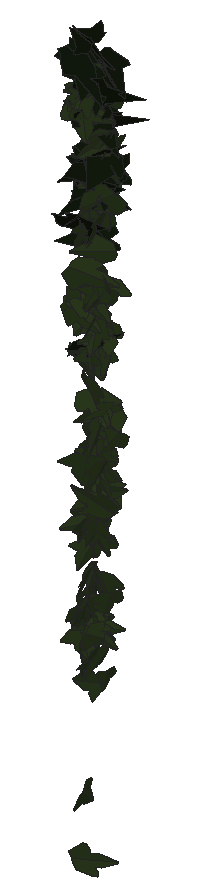
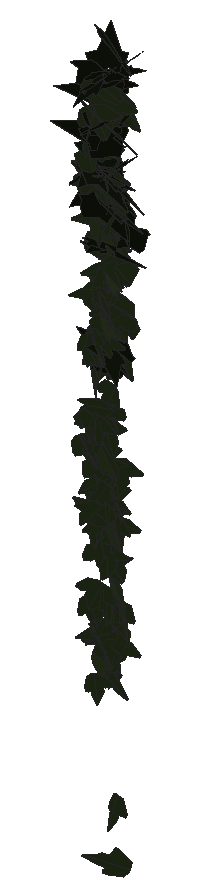
# SketchUp Ruby script. Lengths in inches.
U = 1.inch
M = Sketchup.active_model
def pt(a) = Geom::Point3d.new(a.map { |v| v * U })
def face(e, loops, mat)
  f = e.add_face(loops[0].map { |a| pt(a) })
  loops[1..].each { |l| e.add_face(l.map { |a| pt(a) }).erase! }
  f.material = f.back_material = mat if mat
  f
end
# faces: each face lists its corners as indices into pts; further lists are holes
def faces(e, pts, list, mat = nil) = list.each { |f| face(e, (f[0].is_a?(Array) ? f : [f]).map { |l| l.map { |i| pts[i] } }, mat) }
# xy, xz, yz: faces in a plane at the given z, y or x. An outline is a flat list of corners, or four numbers for a rectangle; further outlines are holes
def ring(l) = l.size == 4 ? [[l[0], l[1]], [l[2], l[1]], [l[2], l[3]], [l[0], l[3]]] : l.each_slice(2).to_a
def flat(e, list, mat, &to3) = list.each { |f| face(e, (f[0].is_a?(Array) ? f : [f]).map { |l| ring(l).map { |u, v| to3.(u, v) } }, mat) }
def xy(e, z, list, mat = nil) = flat(e, list, mat) { |x, y| [x, y, z] }
def xz(e, y, list, mat = nil) = flat(e, list, mat) { |x, z| [x, y, z] }
def yz(e, x, list, mat = nil) = flat(e, list, mat) { |y, z| [x, y, z] }
def lines(e, pts, list) = list.each { |a, b| e.add_line(pt(pts[a]), pt(pts[b])) }
# prism: a flat outline (further loops are holes) pulled along v
def prism(e, loops, v, mat = nil)
  f = face(e, loops, mat); d = Geom::Vector3d.new(v.map { |x| x * U })
  f.pushpull(f.normal.samedirection?(d) ? d.length : -d.length)
end
def box(e, o, s, mat = nil) = prism(e, [[o, [o[0] + s[0], o[1], o[2]], [o[0] + s[0], o[1] + s[1], o[2]], [o[0], o[1] + s[1], o[2]]]], [0, 0, s[2]], mat)
def at(x, y, z, deg = 0) = Geom::Transformation.translation(pt([x, y, z])) * Geom::Transformation.rotation(ORIGIN, Z_AXIS, deg.degrees)
def axes(o, x, y, z) = Geom::Transformation.new([*x, 0, *y, 0, *z, 0, *pt(o).to_a, 1])
def part(name) = M.definitions.add(name)
# library, detail: a bought-in or finely detailed component or shape, given as its bounding box
def library(name, o, s) = part(name).tap { |d| box(d.entities, o, s) }
def detail(e, o, s) = box(e.add_group.entities, o, s)
def put(e, d, t, mat = nil) = e.add_instance(d, t).tap { |i| i.material = mat if mat }
def group(e, t, mat = nil) = e.add_group.tap { |g| g.transformation = t; g.material = mat if mat }.entities
root = M.entities
M.materials.add("1026 AP 7946 SUNNY SIDE UP").color = [254, 231, 186]
M.materials.add("efeu1").color = [18, 25, 13]
M.materials.add("efeu2").color = [43, 57, 29]
c1 = part("ivyleaf_10")
p = [[0,0.5,-0.03],[-0.0625,2.02,-0.43],[-0.19,2.01,-0.46],[-0.54,1.05,-0.29],[-0.52,0.625,-0.18],[-0.83,0.76,-0.28],
  [-1.16,0.64,-0.33],[-1.15,0.33,-0.24],[-0.77,-0.39,0.02],[-0.3,-0.51,0.16],[0.04,-0.48,0.23],[-0.02,2.01,-0.4375],
  [-0.06,2.01,-0.43],[0.04,-0.49,0.23],[0.67,-0.49,0.14],[1.38,0.36,-0.2],[1.375,0.51,-0.24],[0.81,0.65,-0.19],
  [0.62,0.59,-0.15],[0.6,1.09,-0.28],[0.5,1.23,-0.31]]
faces(c1.entities,p,[[0,1,2,3,4,5,6,7,8,9,10],[11,12,0,13,14,15,16,17,18,19,20]],"efeu2")
c2 = part("ivyleaf_9")
p = [[1.54,2.16,1.25],[1.36,2.04,1.19],[-0.21,0.99,0.68],[-0.71,1.11,0.82],[-0.85,0.86,0.67],[-0.8,0.17,0.21],
  [-0.9,-0.01,0.1],[-0.67,-0.16,-0.02],[-0.08,-0.08,-0.05],[-0.03,-0.6,-0.4],[0.65,-0.88,-0.66],[0.83,-0.6,-0.49],
  [1.29,-0.42,-0.43],[1.8125,-0.07,-0.26],[1.21,0.44,0.15]]
faces(c2.entities,p,[[0,1,2,3,4,5,6,7,8,9,10,11,12,13,14]],"efeu1")
put(root,c1,axes([99.3125,212.71,264.43],[-0.12785,0.21743,0.05736],[-0.07153,0.0407,-0.23721],[-0.3451,-0.08899,0.02792]),"1026 AP 7946 SUNNY SIDE UP")
put(root,c1,axes([99.32,212.63,257.54],[0.10302,-0.18844,-0.06794],[-0.02315,0.06353,-0.20504],[0.31252,0.06682,0.0072]),"1026 AP 7946 SUNNY SIDE UP")
put(root,c1,axes([99.4,212.64,266.76],[0.25779,-0.12483,-0.10927],[-0.15343,0.04752,-0.20886],[0.22457,0.17576,-0.01726]),"1026 AP 7946 SUNNY SIDE UP")
put(root,c1,axes([99.25,212.95,264.75],[-0.09069,0.23059,-0.04473],[0.00337,-0.04554,-0.24497],[-0.36932,-0.05704,0.00875]),"1026 AP 7946 SUNNY SIDE UP")
put(root,c1,axes([99.33,212.89,258.47],[-0.11329,-0.16436,0.10325],[0.01129,-0.11018,-0.17981],[0.30326,-0.0573,0.04527]),"1026 AP 7946 SUNNY SIDE UP")
put(root,c2,axes([99.49,212.85,265.46],[-0.29653,0.15424,-0.02154],[0.00846,-0.02773,-0.25046],[-0.24478,-0.1878,0.01743]),"1026 AP 7946 SUNNY SIDE UP")
put(root,c2,axes([99.49,212.71,267.73],[-0.08229,0.16878,0.1343],[-0.09177,0.11209,-0.18553],[-0.34269,-0.07054,0.01743]),"1026 AP 7946 SUNNY SIDE UP")
put(root,c1,axes([99.32,212.84,265.11],[-0.32117,0.13465,-0.01253],[0.00024,-0.02319,-0.25138],[-0.2127,-0.20334,0.01864]),"1026 AP 7946 SUNNY SIDE UP")
put(root,c1,axes([99.36,212.89,266.77],[-0.26787,-0.14859,-0.00001],[0.01642,-0.01308,-0.23158],[0.25172,-0.15727,0.0151]),"1026 AP 7946 SUNNY SIDE UP")
put(root,c1,axes([99.3,212.78,265.62],[-0.10561,0.19686,0.0015],[-0.00787,-0.00268,-0.22099],[-0.33409,-0.06217,0.00473]),"1026 AP 7946 SUNNY SIDE UP")
put(root,c2,axes([99.48,212.9,264.98],[-0.32998,0.09373,-0.07749],[0.06939,-0.08177,-0.23067],[-0.17633,-0.20759,0.05423]),"1026 AP 7946 SUNNY SIDE UP")
put(root,c1,axes([99.29,212.72,262.05],[-0.30133,0.06326,-0.05947],[0.07549,-0.04183,-0.20076],[-0.12243,-0.18149,0.02257]),"1026 AP 7946 SUNNY SIDE UP")
put(root,c2,axes([99.15,212.6,264.46],[0.38988,0.04482,0.02646],[0.04087,0.0026,-0.25048],[-0.07614,0.23092,0.00103]),"1026 AP 7946 SUNNY SIDE UP")
put(root,c1,axes([99.35,212.72,254.09],[-0.01126,-0.16253,-0.15866],[0.03044,0.15214,-0.16644],[0.34975,-0.01847,0.00938]),"1026 AP 7946 SUNNY SIDE UP")
put(root,c2,axes([99.47,212.83,262.31],[-0.00226,0.20899,0.05213],[-0.04174,0.04552,-0.22166],[-0.36085,-0.00658,0.02532]),"1026 AP 7946 SUNNY SIDE UP")
put(root,c2,axes([99.31,212.94,267.34],[-0.18447,-0.22711,-0.003],[0.01421,-0.00284,-0.26318],[0.35683,-0.11729,0.00893]),"1026 AP 7946 SUNNY SIDE UP")
put(root,c1,axes([99.3,213.27,264.55],[-0.00588,-0.08446,-0.1888],[0.00093,-0.17528,0.08798],[-0.33024,0.00101,0.00361]),"1026 AP 7946 SUNNY SIDE UP")
put(root,c1,axes([99.38,212.8125,264.35],[0.0144,-0.22414,0.09343],[0.00479,-0.09191,-0.23164],[0.38092,0.00963,-0.00062]),"1026 AP 7946 SUNNY SIDE UP")
put(root,c2,axes([99.61,212.97,266.53],[-0.24542,0.17282,0.09286],[-0.12348,0.04857,-0.23834],[-0.27973,-0.17307,0.02374]),"1026 AP 7946 SUNNY SIDE UP")
put(root,c1,axes([99.4,212.72,260.12],[-0.26726,-0.16108,0.0194],[-0.00401,-0.02594,-0.24075],[0.25514,-0.16913,0.01654]),"1026 AP 7946 SUNNY SIDE UP")
put(root,c2,axes([99.47,212.95,265.06],[-0.01462,0.19554,-0.14762],[-0.00865,-0.14464,-0.20225],[-0.38212,-0.00421,0.01022]),"1026 AP 7946 SUNNY SIDE UP")
put(root,c1,axes([99.4,212.92,260.89],[-0.07265,-0.21475,0.01095],[-0.00438,-0.01152,-0.22636],[0.33816,-0.04629,-0.00058]),"1026 AP 7946 SUNNY SIDE UP")
put(root,c1,axes([99.32,212.71,256.91],[-0.23853,-0.11981,-0.03131],[0.10214,-0.03034,-0.18685],[0.18204,-0.13997,0.06382]),"1026 AP 7946 SUNNY SIDE UP")
put(root,c1,axes([99.45,212.85,262.79],[-0.24276,-0.11438,0.13264],[-0.05924,-0.14708,-0.1811],[0.26502,-0.13765,0.08101]),"1026 AP 7946 SUNNY SIDE UP")
put(root,c1,axes([99.4,212.93,260.42],[0.00099,-0.20825,0.0585],[-0.00089,-0.05797,-0.21488],[0.33991,0.00045,-0.00073]),"1026 AP 7946 SUNNY SIDE UP")
put(root,c1,axes([99.38,212.75,258.05],[0.12663,-0.21232,0.04084],[0.01364,-0.04038,-0.23409],[0.33971,0.08077,-0.00583]),"1026 AP 7946 SUNNY SIDE UP")
put(root,c1,axes([99.33,212.7,256.66],[-0.04075,0.16326,-0.06769],[0.01296,-0.06494,-0.17756],[-0.29824,-0.02513,0.00154]),"1026 AP 7946 SUNNY SIDE UP")
put(root,c1,axes([99.16,212.7,262.84],[-0.17306,-0.03078,-0.20882],[0.28399,-0.12307,-0.08256],[-0.152,-0.19489,0.08349]),"1026 AP 7946 SUNNY SIDE UP")
put(root,c1,axes([99.37,212.95,262.89],[0.08664,-0.20923,0.12729],[0.04852,-0.12087,-0.2236],[0.37994,0.06315,-0.00047]),"1026 AP 7946 SUNNY SIDE UP")
put(root,c1,axes([99.47,212.98,265.47],[-0.3396,-0.08304,0.04682],[-0.06092,-0.03021,-0.23184],[0.14814,-0.20277,0.012]),"1026 AP 7946 SUNNY SIDE UP")
put(root,c1,axes([99.41,212.72,259.03],[0.02325,-0.21147,0.01885],[0.00075,-0.01951,-0.2185],[0.33392,0.01477,-0.00082]),"1026 AP 7946 SUNNY SIDE UP")
put(root,c1,axes([99.46,212.94,258.68],[-0.28355,-0.08817,0.04329],[-0.04474,-0.03806,-0.20585],[0.14726,-0.18132,0.02081]),"1026 AP 7946 SUNNY SIDE UP")
put(root,c1,axes([99.38,212.95,264.9],[-0.18415,0.21231,-0.00502],[-0.02109,-0.01433,-0.24913],[-0.3333,-0.11639,0.01854]),"1026 AP 7946 SUNNY SIDE UP")
put(root,c2,axes([99.22,212.69,267.4],[0.11181,-0.24319,-0.05237],[0.00191,0.05179,-0.26024],[0.39021,0.06943,0.01628]),"1026 AP 7946 SUNNY SIDE UP")
put(root,c1,axes([99.36,212.88,263.63],[0.11453,-0.1524,0.12885],[0.0613,-0.11748,-0.17963],[0.32603,0.07562,-0.01149]),"1026 AP 7946 SUNNY SIDE UP")
put(root,c1,axes([99.43,212.58,259.32],[0.12383,-0.19006,-0.0699],[-0.02234,0.06628,-0.21121],[0.31596,0.07917,0.01246]),"1026 AP 7946 SUNNY SIDE UP")
put(root,c2,axes([99.4375,212.8125,265.375],[-0.13107,-0.07483,0.1929],[-0.1236,-0.16983,-0.11069],[0.30892,-0.0997,0.03756]),"1026 AP 7946 SUNNY SIDE UP")
put(root,c2,axes([99.58,212.94,265.58],[-0.13863,0.22233,-0.05674],[-0.0252,-0.06619,-0.24361],[-0.35976,-0.08104,0.03893]),"1026 AP 7946 SUNNY SIDE UP")
put(root,c1,axes([99.56,212.73,259.08],[-0.08607,-0.04117,0.2176],[-0.16013,-0.18731,-0.06582],[0.29849,-0.11235,0.02743]),"1026 AP 7946 SUNNY SIDE UP")
put(root,c2,axes([99.65,212.94,264.14],[-0.31806,0.02914,0.09731],[-0.15861,-0.01928,-0.20068],[-0.02997,-0.20718,0.02939]),"1026 AP 7946 SUNNY SIDE UP")
put(root,c1,axes([99.42,212.87,257.83],[-0.01359,-0.20294,-0.04341],[0.02623,0.0402,-0.20848],[0.32449,-0.01175,0.01504]),"1026 AP 7946 SUNNY SIDE UP")
put(root,c1,axes([99.4,212.8,261.51],[-0.25527,0.11699,-0.01699],[0.00854,-0.02179,-0.20372],[-0.20059,-0.1498,0.01295]),"1026 AP 7946 SUNNY SIDE UP")
put(root,c1,axes([99.5,213.07,266.6],[-0.24073,-0.13764,0.06163],[-0.05168,-0.05357,-0.21158],[0.24915,-0.1441,0.01566]),"1026 AP 7946 SUNNY SIDE UP")
put(root,c1,axes([99.5625,212.97,267.07],[-0.19589,-0.09439,0.16139],[-0.1463,-0.12916,-0.15774],[0.26615,-0.14047,0.03208]),"1026 AP 7946 SUNNY SIDE UP")
put(root,c1,axes([99.34,212.93,265.08],[-0.33974,0.04005,-0.10864],[0.10889,-0.13328,-0.19867],[-0.14045,-0.20023,0.10877]),"1026 AP 7946 SUNNY SIDE UP")
put(root,c2,axes([99.53,212.51,264.76],[-0.03765,0.21506,0.00773],[0.00302,0.00462,-0.23138],[-0.36514,-0.02214,-0.00271]),"1026 AP 7946 SUNNY SIDE UP")
put(root,c1,axes([99.43,212.8,259.26],[0.16574,-0.18597,-0.00834],[-0.01553,0.00249,-0.22007],[0.29221,0.10561,-0.00696]),"1026 AP 7946 SUNNY SIDE UP")
put(root,c1,axes([99.21,212.82,262.93],[0.28263,0.07441,0.13929],[0.20418,0.03807,-0.19981],[-0.13008,0.22142,-0.01098]),"1026 AP 7946 SUNNY SIDE UP")
put(root,c1,axes([99.48,212.89,259.73],[0.17606,-0.12454,-0.14214],[-0.07627,0.13509,-0.16623],[0.28128,0.11458,0.04389]),"1026 AP 7946 SUNNY SIDE UP")
put(root,c2,axes([99.36,212.93,266.1],[0.21685,0.14287,0.12944],[-0.18807,-0.05754,0.20039],[0.25356,-0.16486,0.03793]),"1026 AP 7946 SUNNY SIDE UP")
put(root,c1,axes([99.39,212.58,257.51],[-0.117,-0.14835,-0.1356],[0.1024,0.11356,-0.1702],[0.29362,-0.09872,0.00533]),"1026 AP 7946 SUNNY SIDE UP")
put(root,c1,axes([99.45,212.98,262.14],[-0.16059,0.17136,0.02287],[-0.05363,0.00423,-0.20771],[-0.28774,-0.09642,0.02594]),"1026 AP 7946 SUNNY SIDE UP")
put(root,c1,axes([99.68,212.9,264.62],[-0.10826,0.06355,0.19199],[-0.31818,0.00644,-0.07405],[-0.04713,-0.18944,0.05894]),"1026 AP 7946 SUNNY SIDE UP")
put(root,c2,axes([99.32,212.95,267.47],[0.30953,-0.13908,-0.03751],[0.06428,-0.00495,0.24462],[-0.23407,-0.18528,0.01757]),"1026 AP 7946 SUNNY SIDE UP")
put(root,c2,axes([99.37,212.95,267.1],[-0.13954,-0.21284,-0.03908],[0.03591,0.02795,-0.24366],[0.36405,-0.08434,0.00906]),"1026 AP 7946 SUNNY SIDE UP")
put(root,c1,axes([99.47,212.94,263.22],[0.18991,-0.19322,-0.05543],[-0.02726,0.05123,-0.23411],[0.31374,0.12141,0.01321]),"1026 AP 7946 SUNNY SIDE UP")
put(root,c1,axes([99.39,212.67,257.43],[-0.05825,-0.11153,-0.20819],[0.12646,0.18493,-0.11962],[0.33927,-0.08808,0.00885]),"1026 AP 7946 SUNNY SIDE UP")
put(root,c2,axes([99.26,212.74,262.07],[0.21178,0.17457,-0.03492],[0.00398,0.04099,0.22911],[0.30218,-0.12289,0.02145]),"1026 AP 7946 SUNNY SIDE UP")
put(root,c2,axes([99.4,212.88,266.33],[0.17775,0.15261,0.16346],[-0.19038,-0.10471,0.19307],[0.28794,-0.16345,0.02675]),"1026 AP 7946 SUNNY SIDE UP")
put(root,c2,axes([99.54,212.91,265.43],[-0.36902,-0.04542,-0.05031],[0.07998,-0.00782,-0.24568],[0.06736,-0.23953,0.0161]),"1026 AP 7946 SUNNY SIDE UP")
put(root,c1,axes([99.3125,212.66,266.47],[0.34185,-0.02066,0.08816],[0.13602,-0.02583,-0.21639],[0.04893,0.21613,-0.01435]),"1026 AP 7946 SUNNY SIDE UP")
put(root,c1,axes([99.4,212.99,259.83],[-0.27358,0.07586,-0.06616],[0.0824,-0.04358,-0.19036],[-0.14544,-0.16738,0.0166]),"1026 AP 7946 SUNNY SIDE UP")
put(root,c1,axes([99.51,213,262.47],[-0.28614,-0.10806,0.0327],[-0.0118,-0.04742,-0.21158],[0.19092,-0.16488,0.03594]),"1026 AP 7946 SUNNY SIDE UP")
put(root,c1,axes([99.52,212.66,259.11],[-0.35805,0.05682,0.03024],[-0.05259,-0.01466,-0.24078],[-0.08544,-0.22908,0.02148]),"1026 AP 7946 SUNNY SIDE UP")
put(root,c1,axes([99.55,212.92,260.21],[-0.22432,-0.13861,0.08679],[-0.04244,-0.09137,-0.20061],[0.25215,-0.13869,0.04344]),"1026 AP 7946 SUNNY SIDE UP")
put(root,c1,axes([99.49,212.73,262.875],[0.13911,0.21918,-0.02212],[0.00077,0.02428,0.24348],[0.34648,-0.08805,0.00834]),"1026 AP 7946 SUNNY SIDE UP")
put(root,c2,axes([99.31,212.94,266.43],[0.05482,-0.24294,-0.10898],[0.01684,0.10652,-0.25104],[0.41544,0.02774,0.02455]),"1026 AP 7946 SUNNY SIDE UP")
put(root,c1,axes([99.48,212.78,265.13],[0.26365,-0.12931,-0.00049],[-0.01504,-0.01256,-0.21592],[0.21901,0.15481,-0.01424]),"1026 AP 7946 SUNNY SIDE UP")
put(root,c2,axes([99.65,212.76,262.37],[-0.22167,0.17066,-0.03037],[0.01201,-0.03302,-0.23],[-0.29407,-0.12999,0.0135]),"1026 AP 7946 SUNNY SIDE UP")
put(root,c1,axes([99.625,213.02,261.11],[-0.18017,-0.0514,0.15454],[-0.14199,-0.12859,-0.11613],[0.21921,-0.12554,0.05179]),"1026 AP 7946 SUNNY SIDE UP")
put(root,c1,axes([99.64,212.58,256.24],[0.13234,-0.06625,-0.17795],[-0.21163,0.10767,-0.10971],[0.19877,0.15874,0.00167]),"1026 AP 7946 SUNNY SIDE UP")
put(root,c1,axes([99.33,212.73,263.15],[-0.2867,-0.04369,-0.14969],[0.24774,-0.05299,-0.17243],[-0.00284,-0.21239,0.07054]),"1026 AP 7946 SUNNY SIDE UP")
put(root,c1,axes([99.5,212.59,257.59],[0.06629,-0.19538,-0.08044],[0.02252,0.081,-0.20326],[0.32943,0.03378,0.03008]),"1026 AP 7946 SUNNY SIDE UP")
put(root,c1,axes([99.64,212.73,259.45],[-0.10828,-0.06411,0.16779],[-0.15312,-0.12992,-0.0975],[0.24483,-0.10961,0.01323]),"1026 AP 7946 SUNNY SIDE UP")
put(root,c1,axes([99.53,212.61,256.62],[0.03247,-0.1823,-0.00129],[-0.0026,-0.00134,-0.19624],[0.30945,0.01912,-0.00152]),"1026 AP 7946 SUNNY SIDE UP")
put(root,c1,axes([99.36,212.73,257.21],[-0.18353,-0.08898,-0.14873],[0.22496,0.04134,-0.14567],[0.14192,-0.18059,0.03857]),"1026 AP 7946 SUNNY SIDE UP")
put(root,c1,axes([99.52,212.74,263.52],[-0.10652,-0.20352,-0.04789],[0.03992,0.03671,-0.22717],[0.35053,-0.06603,0.01132]),"1026 AP 7946 SUNNY SIDE UP")
put(root,c1,axes([99.35,212.65,266.48],[-0.08483,-0.08666,-0.20235],[0.2529,0.11906,-0.09955],[0.24373,-0.1537,0.03286]),"1026 AP 7946 SUNNY SIDE UP")
put(root,c1,axes([99.51,212.56,257.53],[-0.0499,-0.16937,-0.15118],[0.05524,0.14164,-0.17657],[0.34703,-0.0469,0.00637]),"1026 AP 7946 SUNNY SIDE UP")
put(root,c1,axes([99.43,212.9375,263.03],[0.20502,-0.13283,0.10987],[0.11823,-0.07772,-0.19328],[0.26125,0.13942,0.00125]),"1026 AP 7946 SUNNY SIDE UP")
put(root,c1,axes([99.63,212.96,262.49],[0.16375,-0.11588,-0.15578],[-0.12208,0.1261,-0.15846],[0.28905,0.11891,0.02133]),"1026 AP 7946 SUNNY SIDE UP")
put(root,c1,axes([99.62,212.86,265.89],[0.05474,0.08187,-0.19696],[-0.17989,-0.1528,-0.09428],[-0.29262,0.10925,0.02111]),"1026 AP 7946 SUNNY SIDE UP")
put(root,c1,axes([99.57,213,261],[-0.30809,-0.00471,0.01094],[-0.01643,-0.02089,-0.1934],[0.00994,-0.18058,0.01953]),"1026 AP 7946 SUNNY SIDE UP")
put(root,c1,axes([99.37,213.05,259.35],[-0.17168,-0.04535,0.15521],[0.21749,0.06943,0.11942],[-0.14032,0.16309,-0.00481]),"1026 AP 7946 SUNNY SIDE UP")
put(root,c1,axes([99.5625,212.93,262.47],[-0.08784,-0.19243,-0.04522],[0.01971,0.03802,-0.21279],[0.33296,-0.05302,0.00067]),"1026 AP 7946 SUNNY SIDE UP")
put(root,c1,axes([99.7,212.92,264.59],[-0.05569,0.10076,0.17777],[-0.23355,0.10506,-0.09666],[-0.23003,-0.13106,0.0551]),"1026 AP 7946 SUNNY SIDE UP")
put(root,c1,axes([99.58,213,261.05],[-0.11088,0.14892,0.07953],[-0.07588,0.05902,-0.17245],[-0.27061,-0.07757,0.01577]),"1026 AP 7946 SUNNY SIDE UP")
put(root,c2,axes([99.5,212.75,265.65],[0.19776,0.17606,0.12181],[0.07607,0.10884,-0.22121],[-0.32378,0.13311,0.02243]),"1026 AP 7946 SUNNY SIDE UP")
put(root,c2,axes([99.3125,212.92,266.16],[0.14037,0.14852,-0.15928],[0.10664,0.13729,0.18365],[0.34299,-0.10346,0.00809]),"1026 AP 7946 SUNNY SIDE UP")
put(root,c1,axes([99.51,212.82,257.29],[0.0997,-0.08644,-0.18028],[0.08819,0.18385,-0.07174],[0.29323,-0.0259,0.08288]),"1026 AP 7946 SUNNY SIDE UP")
put(root,c1,axes([99.35,212.63,252.9],[-0.06915,-0.00823,0.21019],[0.25165,0.12831,0.04161],[-0.19952,0.16468,-0.02036]),"1026 AP 7946 SUNNY SIDE UP")
put(root,c1,axes([99.46,213.07,259.51],[0.1293,0.14248,0.08975],[0.07353,0.06976,-0.17192],[-0.26919,0.0875,-0.00385]),"1026 AP 7946 SUNNY SIDE UP")
put(root,c1,axes([99.55,212.73,260.8],[0.02426,0.1181,-0.14093],[-0.04266,-0.13093,-0.12901],[-0.29913,0.02825,0.00697]),"1026 AP 7946 SUNNY SIDE UP")
put(root,c1,axes([99.81,212.65,259.42],[-0.19001,0.00731,-0.19564],[-0.29887,-0.0077,0.12422],[-0.00405,0.225,0.01193]),"1026 AP 7946 SUNNY SIDE UP")
put(root,c1,axes([99.54,212.94,257.97],[-0.31333,0.01887,-0.04387],[0.06408,-0.02089,-0.20562],[-0.03577,-0.20272,0.0159]),"1026 AP 7946 SUNNY SIDE UP")
put(root,c1,axes([99.58,212.92,259.1],[0.03012,0.17456,0.04481],[-0.07606,0.04284,-0.18016],[-0.29417,0.00679,0.05117]),"1026 AP 7946 SUNNY SIDE UP")
put(root,c1,axes([99.55,212.93,265.42],[-0.30508,0.14106,-0.0536],[0.03234,-0.06054,-0.24468],[-0.23464,-0.19176,0.03598]),"1026 AP 7946 SUNNY SIDE UP")
put(root,c1,axes([99.62,212.9,265.99],[-0.08641,-0.22058,0.09529],[0.00016,-0.0962,-0.23369],[0.37687,-0.05054,0.02195]),"1026 AP 7946 SUNNY SIDE UP")
put(root,c1,axes([99.51,213.08,265.39],[0.09037,0.18422,0.04216],[0.02534,0.03417,-0.20475],[-0.31796,0.05509,-0.00433]),"1026 AP 7946 SUNNY SIDE UP")
put(root,c1,axes([99.64,212.59,262.875],[0.04679,-0.18637,-0.17383],[-0.03749,0.16599,-0.19344],[0.39241,0.03808,0.00224]),"1026 AP 7946 SUNNY SIDE UP")
put(root,c1,axes([99.6,213.05,262.31],[-0.02311,-0.18262,0.08916],[0.0296,-0.0866,-0.1959],[0.34114,-0.00486,0.02303]),"1026 AP 7946 SUNNY SIDE UP")
put(root,c1,axes([99.69,212.77,263.24],[-0.1847,-0.1462,0.10484],[-0.07857,-0.08961,-0.19575],[0.29007,-0.11736,0.01373]),"1026 AP 7946 SUNNY SIDE UP")
put(root,c1,axes([99.43,212.85,261.22],[0.28286,0.10333,0.08811],[0.13198,0.02364,-0.21261],[-0.16377,0.19753,-0.01916]),"1026 AP 7946 SUNNY SIDE UP")
put(root,c1,axes([99.77,212.74,264.04],[-0.04585,-0.01708,0.21021],[-0.20556,-0.15522,-0.03442],[0.26446,-0.12361,0.00969]),"1026 AP 7946 SUNNY SIDE UP")
put(root,c1,axes([99.42,212.74,257.09],[-0.20843,-0.02379,-0.15648],[0.25011,-0.00512,-0.13197],[0.01929,-0.19058,0.02038]),"1026 AP 7946 SUNNY SIDE UP")
put(root,c1,axes([99.48,212.87,259.9],[0.11305,0.05926,0.16386],[0.09076,0.1475,-0.08442],[-0.26213,0.07663,0.04144]),"1026 AP 7946 SUNNY SIDE UP")
put(root,c1,axes([99.55,212.86,256.86],[0.11092,-0.16449,0.04526],[-0.01525,0.04418,0.18992],[-0.28882,-0.0655,0.00735]),"1026 AP 7946 SUNNY SIDE UP")
put(root,c1,axes([99.61,213.02,266.5],[-0.16168,0.17519,0.03246],[-0.04647,0.01692,-0.21257],[-0.29756,-0.09783,0.01556]),"1026 AP 7946 SUNNY SIDE UP")
put(root,c1,axes([99.42,212.77,264.7],[-0.02505,-0.04484,-0.25449],[0.27296,0.17651,-0.04356],[0.28466,-0.1732,0.01937]),"1026 AP 7946 SUNNY SIDE UP")
put(root,c1,axes([99.55,212.8125,258.86],[-0.26812,0.06876,-0.05697],[0.0702,-0.03973,-0.18385],[-0.13089,-0.16216,0.01808]),"1026 AP 7946 SUNNY SIDE UP")
put(root,c1,axes([99.73,212.86,265.33],[0.17806,0.04427,-0.17203],[-0.22996,-0.08913,-0.12177],[-0.16646,0.17048,-0.0158]),"1026 AP 7946 SUNNY SIDE UP")
put(root,c1,axes([99.6,212.77,262.09],[-0.21343,-0.16685,-0.01041],[0.07222,-0.02285,-0.21807],[0.27416,-0.12386,0.04934]),"1026 AP 7946 SUNNY SIDE UP")
put(root,c2,axes([99.51,212.99,267.22],[0.2704,-0.10784,-0.09873],[-0.13832,0.0414,-0.20506],[0.1953,0.17862,-0.00854]),"1026 AP 7946 SUNNY SIDE UP")
put(root,c1,axes([99.65,212.75,259.05],[-0.01752,-0.19387,0.0867],[-0.01338,-0.0849,-0.20052],[0.33274,-0.01363,-0.0035]),"1026 AP 7946 SUNNY SIDE UP")
put(root,c2,axes([99.45,212.99,267.36],[-0.12737,-0.10799,-0.17745],[0.20164,0.1153,-0.13755],[0.26604,-0.13909,0.0193]),"1026 AP 7946 SUNNY SIDE UP")
put(root,c1,axes([99.64,212.95,261.94],[0.13907,-0.18817,-0.09243],[-0.01625,0.09224,-0.21178],[0.32667,0.08469,0.02882]),"1026 AP 7946 SUNNY SIDE UP")
put(root,c1,axes([99.64,212.89,256.26],[-0.08834,-0.16779,-0.02134],[0.00692,0.01731,-0.18783],[0.28633,-0.05219,-0.00205]),"1026 AP 7946 SUNNY SIDE UP")
put(root,c1,axes([99.4,212.51,263.67],[-0.14512,-0.08984,-0.23302],[0.32123,0.1019,-0.12726],[0.20663,-0.22151,0.03418]),"1026 AP 7946 SUNNY SIDE UP")
put(root,c1,axes([99.61,212.82,264.54],[0.10872,-0.20396,0.10203],[0.03451,-0.09825,-0.22221],[0.35565,0.07188,-0.00963]),"1026 AP 7946 SUNNY SIDE UP")
put(root,c1,axes([99.54,212.7,258.22],[0.16722,-0.13659,0.12026],[0.09887,-0.09974,-0.17864],[0.26551,0.12317,-0.00922]),"1026 AP 7946 SUNNY SIDE UP")
put(root,c1,axes([99.64,212.76,260.07],[0.00968,-0.20481,0.07562],[0.0135,-0.07431,-0.21144],[0.34246,0.00872,0.0062]),"1026 AP 7946 SUNNY SIDE UP")
put(root,c1,axes([99.75,212.8,262.45],[0.08714,0.02451,-0.18917],[-0.2132,-0.12608,-0.05944],[-0.21582,0.13445,-0.01766]),"1026 AP 7946 SUNNY SIDE UP")
put(root,c1,axes([99.59,213.1,265.67],[-0.00908,-0.20358,-0.06928],[-0.00521,-0.062,0.21715],[-0.36125,0.00601,-0.00139]),"1026 AP 7946 SUNNY SIDE UP")
put(root,c1,axes([99.64,212.8,256.65],[0.0452,-0.15409,0.1649],[0.03588,-0.15938,-0.16234],[0.3485,0.0364,-0.00467]),"1026 AP 7946 SUNNY SIDE UP")
put(root,c1,axes([99.65,213.04,260.53],[-0.06563,0.1073,0.14616],[0.02629,-0.13576,0.11826],[0.29172,0.03637,0.02223]),"1026 AP 7946 SUNNY SIDE UP")
put(root,c1,axes([99.8125,212.68,263.35],[-0.02465,-0.00176,-0.20991],[-0.19799,0.1581,0.00993],[0.26753,0.11684,-0.01199]),"1026 AP 7946 SUNNY SIDE UP")
put(root,c1,axes([99.64,212.84,263.22],[0.00642,-0.10075,0.18752],[0.0333,-0.1755,-0.11016],[0.34334,0.0189,0.00718]),"1026 AP 7946 SUNNY SIDE UP")
put(root,c1,axes([99.58,212.77,260.74],[0.01252,-0.13078,0.19238],[0.12654,-0.17398,-0.12957],[0.33643,0.07031,0.04158]),"1026 AP 7946 SUNNY SIDE UP")
put(root,c1,axes([99.79,212.93,261.03],[0.11268,0.04997,-0.18751],[-0.23808,-0.106,-0.09043],[-0.19893,0.15516,0.00201]),"1026 AP 7946 SUNNY SIDE UP")
put(root,c2,axes([99.59,212.99,265.42],[-0.12014,-0.2305,-0.01516],[0.00623,0.01281,-0.25009],[0.363,-0.07651,-0.00073]),"1026 AP 7946 SUNNY SIDE UP")
put(root,c2,axes([99.87,212.97,265.42],[-0.29915,0.15038,0.00697],[-0.02832,-0.01329,-0.24891],[-0.23493,-0.18988,0.02113]),"1026 AP 7946 SUNNY SIDE UP")
put(root,c1,axes([99.7,212.92,257.67],[-0.13239,-0.18345,0.0164],[-0.00137,-0.01825,-0.20793],[0.28969,-0.08392,0.00651]),"1026 AP 7946 SUNNY SIDE UP")
put(root,c1,axes([99.76,212.98,260.57],[-0.18592,-0.13253,0.09845],[-0.07586,-0.08403,-0.18436],[0.26486,-0.1171,0.0163]),"1026 AP 7946 SUNNY SIDE UP")
put(root,c1,axes([99.62,212.98,263.28],[0.23791,0.12245,-0.02818],[-0.01949,-0.02917,-0.19906],[-0.2123,0.1399,-0.01331]),"1026 AP 7946 SUNNY SIDE UP")
put(root,c1,axes([99.89,212.66,265.11],[-0.27481,-0.04855,0.17555],[-0.24395,-0.0745,-0.18592],[0.13546,-0.23266,0.02134]),"1026 AP 7946 SUNNY SIDE UP")
put(root,c2,axes([99.66,212.91,265.68],[-0.16288,-0.20524,0.08704],[-0.04243,-0.0822,-0.237],[0.34712,-0.10636,0.01187]),"1026 AP 7946 SUNNY SIDE UP")
put(root,c2,axes([99.39,212.71,266.78],[0.17994,0.04102,0.20946],[0.33183,0.02215,-0.11837],[-0.06667,0.22095,-0.0238]),"1026 AP 7946 SUNNY SIDE UP")
put(root,c1,axes([99.61,212.66,258.25],[-0.08914,0.15135,-0.07985],[0.03937,-0.07298,-0.17252],[-0.28522,-0.05737,0.00114]),"1026 AP 7946 SUNNY SIDE UP")
put(root,c1,axes([99.59,212.68,262.66],[0.32599,-0.09363,0.06923],[0.07967,-0.05138,-0.23324],[0.16331,0.21196,-0.02441]),"1026 AP 7946 SUNNY SIDE UP")
put(root,c1,axes([99.59,212.58,257.09],[-0.07341,-0.09303,-0.18936],[0.15263,0.15569,-0.10598],[0.28489,-0.10739,0.00798]),"1026 AP 7946 SUNNY SIDE UP")
put(root,c1,axes([99.72,212.58,256.92],[0.03203,-0.20213,-0.07792],[-0.0231,0.07335,-0.20874],[0.33794,0.02417,-0.00688]),"1026 AP 7946 SUNNY SIDE UP")
put(root,c1,axes([99.54,213.09,260.32],[0.1601,-0.13156,-0.09694],[0.10815,-0.06327,0.17185],[-0.24682,-0.11306,0.01242]),"1026 AP 7946 SUNNY SIDE UP")
put(root,c2,axes([99.5,212.7,265.16],[0.32879,0.07385,0.04372],[0.0745,-0.00363,-0.22107],[-0.12144,0.19772,-0.01724]),"1026 AP 7946 SUNNY SIDE UP")
put(root,c1,axes([99.53,212.72,257.18],[-0.02065,-0.07725,-0.20914],[0.22426,0.14977,-0.06749],[0.25675,-0.13703,0.04213]),"1026 AP 7946 SUNNY SIDE UP")
